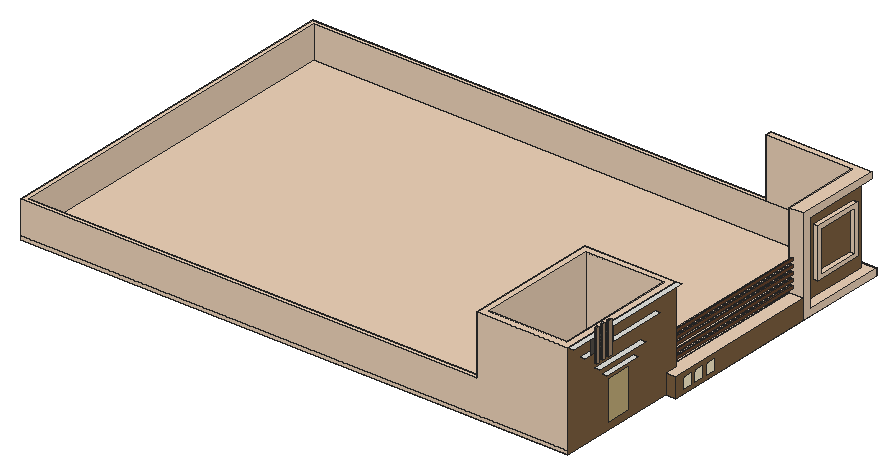
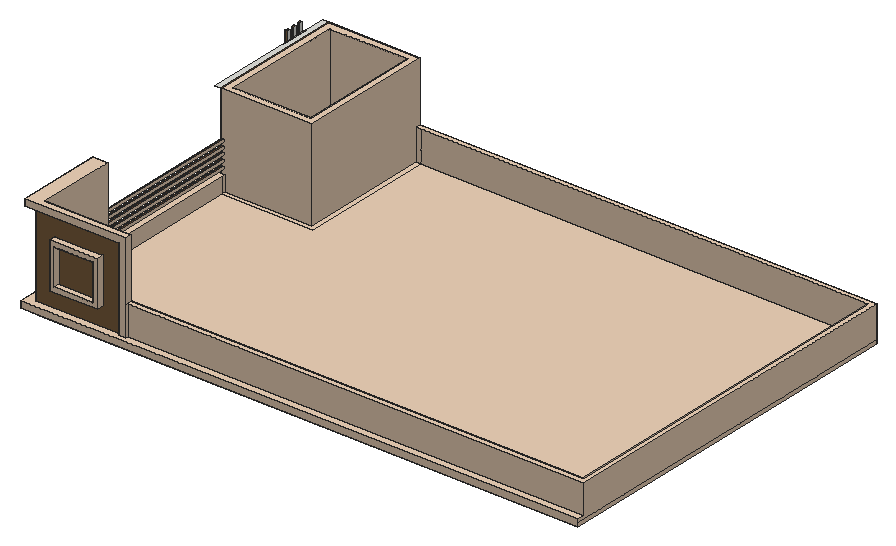
# SketchUp Ruby script. Lengths in inches.
U = 1.inch
M = Sketchup.active_model
def pt(a) = Geom::Point3d.new(a.map { |v| v * U })
def face(e, loops, mat)
  f = e.add_face(loops[0].map { |a| pt(a) })
  loops[1..].each { |l| e.add_face(l.map { |a| pt(a) }).erase! }
  f.material = f.back_material = mat if mat
  f
end
# faces: each face lists its corners as indices into pts; further lists are holes
def faces(e, pts, list, mat = nil) = list.each { |f| face(e, (f[0].is_a?(Array) ? f : [f]).map { |l| l.map { |i| pts[i] } }, mat) }
# xy, xz, yz: faces in a plane at the given z, y or x. An outline is a flat list of corners, or four numbers for a rectangle; further outlines are holes
def ring(l) = l.size == 4 ? [[l[0], l[1]], [l[2], l[1]], [l[2], l[3]], [l[0], l[3]]] : l.each_slice(2).to_a
def flat(e, list, mat, &to3) = list.each { |f| face(e, (f[0].is_a?(Array) ? f : [f]).map { |l| ring(l).map { |u, v| to3.(u, v) } }, mat) }
def xy(e, z, list, mat = nil) = flat(e, list, mat) { |x, y| [x, y, z] }
def xz(e, y, list, mat = nil) = flat(e, list, mat) { |x, z| [x, y, z] }
def yz(e, x, list, mat = nil) = flat(e, list, mat) { |y, z| [x, y, z] }
def lines(e, pts, list) = list.each { |a, b| e.add_line(pt(pts[a]), pt(pts[b])) }
# prism: a flat outline (further loops are holes) pulled along v
def prism(e, loops, v, mat = nil)
  f = face(e, loops, mat); d = Geom::Vector3d.new(v.map { |x| x * U })
  f.pushpull(f.normal.samedirection?(d) ? d.length : -d.length)
end
def box(e, o, s, mat = nil) = prism(e, [[o, [o[0] + s[0], o[1], o[2]], [o[0] + s[0], o[1] + s[1], o[2]], [o[0], o[1] + s[1], o[2]]]], [0, 0, s[2]], mat)
def at(x, y, z, deg = 0) = Geom::Transformation.translation(pt([x, y, z])) * Geom::Transformation.rotation(ORIGIN, Z_AXIS, deg.degrees)
def axes(o, x, y, z) = Geom::Transformation.new([*x, 0, *y, 0, *z, 0, *pt(o).to_a, 1])
def part(name) = M.definitions.add(name)
# library, detail: a bought-in or finely detailed component or shape, given as its bounding box
def library(name, o, s) = part(name).tap { |d| box(d.entities, o, s) }
def detail(e, o, s) = box(e.add_group.entities, o, s)
def put(e, d, t, mat = nil) = e.add_instance(d, t).tap { |i| i.material = mat if mat }
def group(e, t, mat = nil) = e.add_group.tap { |g| g.transformation = t; g.material = mat if mat }.entities
root = M.entities
M.materials.add("D01_Frost_White").color = [255, 242, 206]
M.materials.add("Metal_10_1K").color = [196, 175, 123]
M.materials.add("Plywood_01_1K").color = [125, 96, 64]
M.materials.add("Roofing_01_1K").color = [84, 79, 73]
M.materials.add("ThomThom - Beard1").color = [168, 140, 112]
M.materials.add("ThomThom - Complexion1").color = [237, 210, 184]
M.materials.add("Wood_Veneer_15_1K").color = [103, 69, 45]
c1 = library("Sphere Light\#5",[-2.19,-2.19,-2.19],[4.38,4.38,4.38])
c2 = library("Sphere Light\#3",[-2.0625,-2.0625,-2.0625],[4.125,4.125,4.125])
c3 = library("Sphere Light\#4",[-1.85,-1.85,-1.85],[3.7,3.7,3.7])
xy(root,298,[[0,0,0,489.76,708,489.76,708,480,615,480,615,177,720,177,720,471,733.2,471,733.2,160.5,720,160.5,720,0],[[615,177,615,480,708,480,708,471,720,471,720,177],[705.14,198.45,705.92,198.54,706.65,198.83,707.28,199.29,707.77,199.91,708.08,200.625,708.19,201.4,708.1,202.18,707.82,202.91,707.35,203.53,706.74,204.02,706.02,204.33,705.24,204.45,704.47,204.36,703.74,204.07,703.11,203.61,702.62,202.99,702.31,202.27,702.19,201.5,702.28,200.72,702.57,199.99,703.04,199.36,703.65,198.875,704.37,198.56],[642.95,198.45,643.73,198.54,644.46,198.83,645.09,199.29,645.58,199.91,645.89,200.625,646,201.4,645.92,202.18,645.63,202.91,645.16,203.53,644.55,204.02,643.83,204.33,643.06,204.45,642.28,204.36,641.55,204.07,640.92,203.61,640.43,202.99,640.12,202.27,640.01,201.5,640.09,200.72,640.38,199.99,640.85,199.36,641.46,198.875,642.18,198.56],[705.14,325.42,705.92,325.51,706.65,325.8,707.28,326.27,707.77,326.88,708.08,327.6,708.19,328.37,708.1,329.15,707.82,329.88,707.35,330.51,706.74,330.99,706.02,331.31,705.24,331.42,704.47,331.33,703.74,331.05,703.11,330.58,702.62,329.97,702.31,329.25,702.19,328.47,702.28,327.69,702.57,326.97,703.04,326.34,703.65,325.85,704.37,325.54],[705.14,448.71,705.92,448.8,706.65,449.08,707.28,449.55,707.77,450.16,708.08,450.88,708.19,451.66,708.1,452.43,707.82,453.16,707.35,453.79,706.74,454.28,706.02,454.59,705.24,454.71,704.47,454.62,703.74,454.33,703.11,453.86,702.62,453.25,702.31,452.53,702.19,451.76,702.28,450.98,702.57,450.25,703.04,449.62,703.65,449.13,704.37,448.82],[642.77,448.71,643.55,448.8,644.28,449.08,644.9,449.55,645.39,450.16,645.7,450.88,645.82,451.66,645.73,452.43,645.44,453.16,644.98,453.79,644.36,454.28,643.64,454.59,642.87,454.71,642.09,454.62,641.36,454.33,640.73,453.86,640.25,453.25,639.93,452.53,639.82,451.76,639.91,450.98,640.2,450.25,640.66,449.62,641.28,449.13,641.99,448.82],[642.77,325.42,643.55,325.51,644.28,325.8,644.9,326.27,645.39,326.88,645.7,327.6,645.82,328.37,645.73,329.15,645.44,329.88,644.98,330.51,644.36,330.99,643.64,331.31,642.87,331.42,642.09,331.33,641.36,331.05,640.73,330.58,640.25,329.97,639.93,329.25,639.82,328.47,639.91,327.69,640.2,326.97,640.66,326.34,641.28,325.85,641.99,325.54]],[708,471,720,480],[720,471,733.2,489.76],[708,480,720,489.76]],"ThomThom - Complexion1")
xy(root,299.82,[[642.77,325.42,641.99,325.54,641.28,325.85,640.66,326.34,640.2,326.97,639.91,327.69,639.82,328.47,639.93,329.25,640.25,329.97,640.73,330.58,641.36,331.05,642.09,331.33,642.87,331.42,643.64,331.31,644.36,330.99,644.98,330.51,645.44,329.88,645.73,329.15,645.82,328.37,645.7,327.6,645.39,326.88,644.9,326.27,644.28,325.8,643.55,325.51],[705.14,325.42,704.37,325.54,703.65,325.85,703.04,326.34,702.57,326.97,702.28,327.69,702.19,328.47,702.31,329.25,702.62,329.97,703.11,330.58,703.74,331.05,704.47,331.33,705.24,331.42,706.02,331.31,706.74,330.99,707.35,330.51,707.82,329.88,708.1,329.15,708.19,328.37,708.08,327.6,707.77,326.88,707.28,326.27,706.65,325.8,705.92,325.51],[642.77,448.71,641.99,448.82,641.28,449.13,640.66,449.62,640.2,450.25,639.91,450.98,639.82,451.76,639.93,452.53,640.25,453.25,640.73,453.86,641.36,454.33,642.09,454.62,642.87,454.71,643.64,454.59,644.36,454.28,644.98,453.79,645.44,453.16,645.73,452.43,645.82,451.66,645.7,450.88,645.39,450.16,644.9,449.55,644.28,449.08,643.55,448.8],[705.14,448.71,704.37,448.82,703.65,449.13,703.04,449.62,702.57,450.25,702.28,450.98,702.19,451.76,702.31,452.53,702.62,453.25,703.11,453.86,703.74,454.33,704.47,454.62,705.24,454.71,706.02,454.59,706.74,454.28,707.35,453.79,707.82,453.16,708.1,452.43,708.19,451.66,708.08,450.88,707.77,450.16,707.28,449.55,706.65,449.08,705.92,448.8]],"ThomThom - Complexion1")
xy(root,299.97,[[642.95,198.45,642.18,198.56,641.46,198.875,640.85,199.36,640.38,199.99,640.09,200.72,640.01,201.5,640.12,202.27,640.43,202.99,640.92,203.61,641.55,204.07,642.28,204.36,643.06,204.45,643.83,204.33,644.55,204.02,645.16,203.53,645.63,202.91,645.92,202.18,646,201.4,645.89,200.625,645.58,199.91,645.09,199.29,644.46,198.83,643.73,198.54]],"ThomThom - Complexion1")
xy(root,300.15,[[705.14,198.45,704.37,198.56,703.65,198.875,703.04,199.36,702.57,199.99,702.28,200.72,702.19,201.5,702.31,202.27,702.62,202.99,703.11,203.61,703.74,204.07,704.47,204.36,705.24,204.45,706.02,204.33,706.74,204.02,707.35,203.53,707.82,202.91,708.1,202.18,708.19,201.4,708.08,200.625,707.77,199.91,707.28,199.29,706.65,198.83,705.92,198.54]],"ThomThom - Complexion1")
xy(root,304,[[6,6,594,6,594,183,714,183,714,474,6,474],[594,6,600,6,600,177,714,177,714,183,594,183],[609,9,711,168]],"ThomThom - Complexion1")
xy(root,307,[[720,379.83,733.2,379.83,733.2,489.76,0,489.76,0,480,600,480,600,483,609,483,609,480,720,480]],"ThomThom - Complexion1")
xy(root,324.11,[[720,160.5,733.2,160.5,733.2,370.83,714,370.83,714,177,720,177]],"ThomThom - Complexion1")
xy(root,329.0625,[[720,401.89,727.15,466.9375]],"ThomThom - Complexion1")
xy(root,330.42,[[715.7,170.9375,718.66,370.83]],"ThomThom - Complexion1")
xy(root,331,[[633,480,696,488.28]],"ThomThom - Complexion1")
xy(root,333.95,[[715.7,170.9375,718.66,370.83]],"Wood_Veneer_15_1K")
xy(root,334,[[720,406.83,727.15,462]],"ThomThom - Complexion1")
xy(root,337,[[639,480,690,488.28]],"ThomThom - Complexion1")
xy(root,338.27,[[715.7,170.9375,718.66,370.83]],"ThomThom - Complexion1")
xy(root,341.81,[[715.7,170.9375,718.66,370.83]],"Wood_Veneer_15_1K")
xy(root,346,[[0,0,600,0,600,6,6,6,6,474,600,474,600,480,0,480]],"ThomThom - Complexion1")
xy(root,346.62,[[715.7,170.9375,718.66,370.83]],"ThomThom - Complexion1")
xy(root,350.15,[[715.7,170.9375,718.66,370.83]],"Wood_Veneer_15_1K")
xy(root,354.49,[[715.7,170.9375,718.66,370.83]],"ThomThom - Complexion1")
xy(root,358.02,[[715.7,170.9375,718.66,370.83]],"Wood_Veneer_15_1K")
xy(root,362.31,[[715.7,170.9375,718.66,370.83]],"ThomThom - Complexion1")
xy(root,365.84,[[715.7,170.9375,718.66,370.83]],"Wood_Veneer_15_1K")
xy(root,370,[[722,54,728,105]])
xy(root,382,[[722,42,728,117]])
xy(root,385,[[639,480,690,488.28]],"ThomThom - Complexion1")
xy(root,388,[[720,406.83,727.15,462]],"ThomThom - Complexion1")
xy(root,391,[[633,480,696,488.28]],"ThomThom - Complexion1")
xy(root,392.9375,[[720,401.89,727.15,466.9375]],"ThomThom - Complexion1")
xy(root,394,[[728,33.04,731,37.39],[728,43.39,731,47.22],[728,53.22,731,57.32]])
xy(root,406,[[722,18,728,141]])
xy(root,415,[[720,379.83,733.2,483],[609,480,720,483]],"ThomThom - Complexion1")
xy(root,424,[[720,0,728,177]])
xy(root,424,[[[600,0,720,177],[609,9,711,168]],[714,370.83,733.2,370.83,733.2,483,600,483,600,474,714,474]],"ThomThom - Complexion1")
xy(root,436,[[728,33.04,731,37.39],[728,43.39,731,47.22],[728,53.22,731,57.32]],"Plywood_01_1K")
xz(root,0,[[0,298,720,302.48],[0,302.48,720,302.48,720,424,600,424,600,346,0,346]],"ThomThom - Complexion1")
xz(root,6,[[6,304,594,346],[594,304,600,346]],"ThomThom - Complexion1")
xz(root,9,[[609,304,711,424]],"ThomThom - Complexion1")
xz(root,33.04,[[728,394,731,436]],"Plywood_01_1K")
xz(root,37.39,[[728,394,731,436]],"Plywood_01_1K")
xz(root,43.39,[[728,394,731,436]],"Plywood_01_1K")
xz(root,47.22,[[728,394,731,436]],"Plywood_01_1K")
xz(root,53.22,[[728,394,731,436]],"Plywood_01_1K")
xz(root,57.32,[[728,394,731,436]],"Plywood_01_1K")
xz(root,160.5,[[720,298,733.2,324.11]],"Plywood_01_1K")
xz(root,168,[[609,304,711,424]],"ThomThom - Complexion1")
xz(root,170.9375,[[715.7,330.42,718.66,333.95],[715.7,338.27,718.66,341.81],[715.7,346.62,718.66,350.15],[715.7,354.49,718.66,358.02],[715.7,362.31,718.66,365.84]],"ThomThom - Complexion1")
xz(root,177,[[600,304,600,424,720,424,720,324.11,714,324.11,714,304]],"ThomThom - Complexion1")
xz(root,370.83,[[[714,324.11,733.2,424],[715.7,362.31,718.66,365.84],[715.7,354.49,718.66,358.02],[715.7,346.62,718.66,350.15],[715.7,338.27,718.66,341.81],[715.7,330.42,718.66,333.95]]],"ThomThom - Complexion1")
xz(root,379.83,[[720,307,733.2,415]],"ThomThom - Complexion1")
xz(root,401.89,[[720,329.0625,727.15,392.9375]],"ThomThom - Complexion1")
xz(root,406.83,[[720,334,727.15,388]],"ThomThom - Complexion1")
xz(root,462,[[720,334,727.15,388]],"ThomThom - Complexion1")
xz(root,466.9375,[[720,329.0625,727.15,392.9375]],"ThomThom - Complexion1")
xz(root,474,[[6,304,714,346],[600,346,714,424]],"ThomThom - Complexion1")
xz(root,480,[[[609,307,720,415],[633,331,696,391]],[639,337,690,385]],"Plywood_01_1K")
xz(root,480,[[0,307,600,346]],"ThomThom - Complexion1")
xz(root,483,[[600,307,600,424,733.2,424,733.2,415,609,415,609,307]],"ThomThom - Complexion1")
xz(root,488.28,[[[633,331,696,391],[639,337,690,385]]],"ThomThom - Complexion1")
xz(root,489.76,[[0,298,733.2,307]],"ThomThom - Complexion1")
yz(root,0,[[0,298,489.76,302.48],[0,302.48,0,346,480,346,480,307,489.76,307,489.76,302.48]],"ThomThom - Complexion1")
yz(root,6,[[6,304,474,346]],"ThomThom - Complexion1")
yz(root,600,[[6,304,6,346,0,346,0,424,177,424,177,304],[480,307,483,346],[474,346,483,424]],"ThomThom - Complexion1")
yz(root,609,[[9,304,168,424],[480,307,483,415]],"ThomThom - Complexion1")
yz(root,633,[[480,331,488.28,391]],"ThomThom - Complexion1")
yz(root,639,[[480,337,488.28,385]],"ThomThom - Complexion1")
yz(root,690,[[480,337,488.28,385]],"ThomThom - Complexion1")
yz(root,696,[[480,331,488.28,391]],"ThomThom - Complexion1")
yz(root,711,[[9,304,168,424]],"ThomThom - Complexion1")
yz(root,714,[[177,304,183,324.11],[183,304,183,324.11,370.83,324.11,370.83,424,474,424,474,304]],"ThomThom - Complexion1")
yz(root,715.7,[[170.9375,330.42,370.83,333.95],[170.9375,338.27,370.83,341.81],[170.9375,346.62,370.83,350.15],[170.9375,354.49,370.83,358.02],[170.9375,362.31,370.83,365.84]],"ThomThom - Complexion1")
yz(root,718.66,[[170.9375,330.42,370.83,333.95],[170.9375,338.27,370.83,341.81],[170.9375,346.62,370.83,350.15],[170.9375,354.49,370.83,358.02],[170.9375,362.31,370.83,365.84]],"Wood_Veneer_15_1K")
yz(root,720,[[0,298,160.5,298,160.5,324.11,177,324.11,177,424,0,424],[[379.83,307,480,415],[401.89,329.0625,466.9375,392.9375]],[406.83,334,462,388]],"Plywood_01_1K")
yz(root,722,[[64,309.5,95,360]],"Metal_10_1K")
yz(root,727.15,[[[401.89,329.0625,466.9375,392.9375],[406.83,334,462,388]]],"ThomThom - Complexion1")
yz(root,728,[[33.04,394,37.39,406],[43.39,394,47.22,406],[53.22,394,57.32,406],[33.04,406,37.39,424],[43.39,406,47.22,424],
  [53.22,406,57.32,424],[33.04,424,37.39,436],[43.39,424,47.22,436],[53.22,424,57.32,436]])
yz(root,728,[[27.04,406,33.04,424],[37.39,406,43.39,424],[47.22,406,53.22,424],[57.32,406,63.32,424]],"Roofing_01_1K")
yz(root,731,[[33.04,394,37.39,436],[43.39,394,47.22,436],[53.22,394,57.32,436]],"ThomThom - Beard1")
yz(root,733.2,[[173.05,303.92,185.15,317.39],[191.37,303.92,203.46,317.39],[210.77,303.92,222.86,317.39]],"D01_Frost_White")
yz(root,733.2,[[[160.5,298,370.83,324.11],[173.05,303.92,185.15,317.39],[191.37,303.92,203.46,317.39],[210.77,303.92,222.86,317.39]]],"Plywood_01_1K")
yz(root,733.2,[[370.83,298,489.76,298,489.76,307,379.83,307,379.83,415,483,415,483,424,370.83,424]],"ThomThom - Complexion1")
p = [[642.95,198.45,298],[642.18,198.56,298],[642.18,198.56,299.97],[642.95,198.45,299.97],[643.73,198.54,298],[643.73,198.54,299.97],
  [705.14,198.45,298],[704.37,198.56,298],[704.37,198.56,300.15],[705.14,198.45,300.15],[705.92,198.54,298],[705.92,198.54,300.15],
  [644.46,198.83,298],[644.46,198.83,299.97],[706.65,198.83,298],[706.65,198.83,300.15],[641.46,198.875,298],[641.46,198.875,299.97],
  [703.65,198.875,298],[703.65,198.875,300.15],[645.09,199.29,298],[645.09,199.29,299.97],[707.28,199.29,298],[707.28,199.29,300.15],
  [640.85,199.36,298],[640.85,199.36,299.97],[703.04,199.36,298],[703.04,199.36,300.15],[645.58,199.91,298],[645.58,199.91,299.97],
  [707.77,199.91,298],[707.77,199.91,300.15],[640.38,199.99,298],[640.38,199.99,299.97],[702.57,199.99,298],[702.57,199.99,300.15],
  [645.89,200.625,298],[645.89,200.625,299.97],[708.08,200.625,298],[708.08,200.625,300.15],[640.09,200.72,298],[640.09,200.72,299.97],
  [702.28,200.72,298],[702.28,200.72,300.15],[646,201.4,298],[646,201.4,299.97],[708.19,201.4,298],[708.19,201.4,300.15],
  [640.01,201.5,298],[640.01,201.5,299.97],[702.19,201.5,298],[702.19,201.5,300.15],[645.92,202.18,298],[645.92,202.18,299.97],
  [708.1,202.18,298],[708.1,202.18,300.15],[640.12,202.27,298],[640.12,202.27,299.97],[702.31,202.27,298],[702.31,202.27,300.15],
  [645.63,202.91,298],[645.63,202.91,299.97],[707.82,202.91,298],[707.82,202.91,300.15],[640.43,202.99,298],[640.43,202.99,299.97],
  [702.62,202.99,298],[702.62,202.99,300.15],[645.16,203.53,298],[645.16,203.53,299.97],[707.35,203.53,298],[707.35,203.53,300.15],
  [640.92,203.61,298],[640.92,203.61,299.97],[703.11,203.61,298],[703.11,203.61,300.15],[644.55,204.02,298],[644.55,204.02,299.97],
  [706.74,204.02,298],[706.74,204.02,300.15],[641.55,204.07,298],[641.55,204.07,299.97],[703.74,204.07,298],[703.74,204.07,300.15],
  [643.83,204.33,298],[643.83,204.33,299.97],[706.02,204.33,298],[706.02,204.33,300.15],[642.28,204.36,298],[642.28,204.36,299.97],
  [704.47,204.36,298],[704.47,204.36,300.15],[643.06,204.45,298],[643.06,204.45,299.97],[705.24,204.45,298],[705.24,204.45,300.15],
  [642.77,325.42,298],[641.99,325.54,298],[641.99,325.54,299.82],[642.77,325.42,299.82],[643.55,325.51,298],[643.55,325.51,299.82],
  [705.14,325.42,298],[704.37,325.54,298],[704.37,325.54,299.82],[705.14,325.42,299.82],[705.92,325.51,298],[705.92,325.51,299.82],
  [641.28,325.85,298],[641.28,325.85,299.82],[644.28,325.8,298],[644.28,325.8,299.82],[703.65,325.85,298],[703.65,325.85,299.82],
  [706.65,325.8,298],[706.65,325.8,299.82],[640.66,326.34,298],[640.66,326.34,299.82],[644.9,326.27,298],[644.9,326.27,299.82],
  [703.04,326.34,298],[703.04,326.34,299.82],[707.28,326.27,298],[707.28,326.27,299.82],[640.2,326.97,298],[640.2,326.97,299.82],
  [645.39,326.88,298],[645.39,326.88,299.82],[702.57,326.97,298],[702.57,326.97,299.82],[707.77,326.88,298],[707.77,326.88,299.82],
  [645.7,327.6,298],[645.7,327.6,299.82],[708.08,327.6,298],[708.08,327.6,299.82],[639.91,327.69,298],[639.91,327.69,299.82],
  [702.28,327.69,298],[702.28,327.69,299.82],[645.82,328.37,298],[645.82,328.37,299.82],[708.19,328.37,298],[708.19,328.37,299.82],
  [639.82,328.47,298],[639.82,328.47,299.82],[702.19,328.47,298],[702.19,328.47,299.82],[645.73,329.15,298],[645.73,329.15,299.82],
  [708.1,329.15,298],[708.1,329.15,299.82],[639.93,329.25,298],[639.93,329.25,299.82],[702.31,329.25,298],[702.31,329.25,299.82],
  [645.44,329.88,298],[645.44,329.88,299.82],[707.82,329.88,298],[707.82,329.88,299.82],[640.25,329.97,298],[640.25,329.97,299.82],
  [702.62,329.97,298],[702.62,329.97,299.82],[644.98,330.51,298],[644.98,330.51,299.82],[707.35,330.51,298],[707.35,330.51,299.82],
  [640.73,330.58,298],[640.73,330.58,299.82],[703.11,330.58,298],[703.11,330.58,299.82],[644.36,330.99,298],[644.36,330.99,299.82],
  [706.74,330.99,298],[706.74,330.99,299.82],[641.36,331.05,298],[641.36,331.05,299.82],[703.74,331.05,298],[703.74,331.05,299.82],
  [642.09,331.33,298],[642.09,331.33,299.82],[643.64,331.31,298],[643.64,331.31,299.82],[704.47,331.33,298],[704.47,331.33,299.82],
  [706.02,331.31,298],[706.02,331.31,299.82],[642.87,331.42,298],[642.87,331.42,299.82],[705.24,331.42,298],[705.24,331.42,299.82],
  [642.77,448.71,298],[641.99,448.82,298],[641.99,448.82,299.82],[642.77,448.71,299.82],[643.55,448.8,298],[643.55,448.8,299.82],
  [705.14,448.71,298],[704.37,448.82,298],[704.37,448.82,299.82],[705.14,448.71,299.82],[705.92,448.8,298],[705.92,448.8,299.82],
  [641.28,449.13,298],[641.28,449.13,299.82],[644.28,449.08,298],[644.28,449.08,299.82],[703.65,449.13,298],[703.65,449.13,299.82],
  [706.65,449.08,298],[706.65,449.08,299.82],[640.66,449.62,298],[640.66,449.62,299.82],[644.9,449.55,298],[644.9,449.55,299.82],
  [703.04,449.62,298],[703.04,449.62,299.82],[707.28,449.55,298],[707.28,449.55,299.82],[645.39,450.16,298],[645.39,450.16,299.82],
  [707.77,450.16,298],[707.77,450.16,299.82],[640.2,450.25,298],[640.2,450.25,299.82],[702.57,450.25,298],[702.57,450.25,299.82],
  [639.91,450.98,298],[639.91,450.98,299.82],[645.7,450.88,298],[645.7,450.88,299.82],[702.28,450.98,298],[702.28,450.98,299.82],
  [708.08,450.88,298],[708.08,450.88,299.82],[645.82,451.66,298],[645.82,451.66,299.82],[708.19,451.66,298],[708.19,451.66,299.82],
  [639.82,451.76,298],[639.82,451.76,299.82],[702.19,451.76,298],[702.19,451.76,299.82],[645.73,452.43,298],[645.73,452.43,299.82],
  [708.1,452.43,298],[708.1,452.43,299.82],[639.93,452.53,298],[639.93,452.53,299.82],[702.31,452.53,298],[702.31,452.53,299.82],
  [645.44,453.16,298],[645.44,453.16,299.82],[707.82,453.16,298],[707.82,453.16,299.82],[640.25,453.25,298],[640.25,453.25,299.82],
  [702.62,453.25,298],[702.62,453.25,299.82],[640.73,453.86,298],[640.73,453.86,299.82],[644.98,453.79,298],[644.98,453.79,299.82],
  [703.11,453.86,298],[703.11,453.86,299.82],[707.35,453.79,298],[707.35,453.79,299.82],[644.36,454.28,298],[644.36,454.28,299.82],
  [706.74,454.28,298],[706.74,454.28,299.82],[641.36,454.33,298],[641.36,454.33,299.82],[703.74,454.33,298],[703.74,454.33,299.82],
  [642.09,454.62,298],[642.09,454.62,299.82],[643.64,454.59,298],[643.64,454.59,299.82],[704.47,454.62,298],[704.47,454.62,299.82],
  [706.02,454.59,298],[706.02,454.59,299.82],[642.87,454.71,298],[642.87,454.71,299.82],[705.24,454.71,298],[705.24,454.71,299.82],
  [720,423.06,302],[720,423.06,298],[714,474,338.18],[714,480,338.18],[714,474,330.3125],[714,480,330.3125],
  [714,474,321.97],[714,480,321.97],[714,474,314.11],[714,480,314.11],[720,471,307],[711,480,313]]
faces(root,p,[[0,1,2,3],[4,0,3,5],[6,7,8,9],[10,6,9,11],[12,4,5,13],[14,10,11,15],[1,16,17,2],[7,18,19,8],
  [20,12,13,21],[22,14,15,23],[16,24,25,17],[18,26,27,19],[28,20,21,29],[30,22,23,31],[24,32,33,25],[26,34,35,27],
  [36,28,29,37],[38,30,31,39],[32,40,41,33],[34,42,43,35],[44,36,37,45],[46,38,39,47],[40,48,49,41],[42,50,51,43],
  [52,44,45,53],[54,46,47,55],[48,56,57,49],[50,58,59,51],[60,52,53,61],[62,54,55,63],[56,64,65,57],[58,66,67,59],
  [68,60,61,69],[70,62,63,71],[64,72,73,65],[66,74,75,67],[76,68,69,77],[78,70,71,79],[72,80,81,73],[74,82,83,75],
  [84,76,77,85],[86,78,79,87],[80,88,89,81],[82,90,91,83],[92,84,85,93],[94,86,87,95],[88,92,93,89],[90,94,95,91],
  [96,97,98,99],[100,96,99,101],[102,103,104,105],[106,102,105,107],[97,108,109,98],[110,100,101,111],[103,112,113,104],[114,106,107,115],
  [108,116,117,109],[118,110,111,119],[112,120,121,113],[122,114,115,123],[116,124,125,117],[126,118,119,127],[120,128,129,121],[130,122,123,131],
  [132,126,127,133],[134,130,131,135],[124,136,137,125],[128,138,139,129],[140,132,133,141],[142,134,135,143],[136,144,145,137],[138,146,147,139],
  [148,140,141,149],[150,142,143,151],[144,152,153,145],[146,154,155,147],[156,148,149,157],[158,150,151,159],[152,160,161,153],[154,162,163,155],
  [164,156,157,165],[166,158,159,167],[160,168,169,161],[162,170,171,163],[172,164,165,173],[174,166,167,175],[168,176,177,169],[170,178,179,171],
  [176,180,181,177],[182,172,173,183],[178,184,185,179],[186,174,175,187],[180,188,189,181],[188,182,183,189],[184,190,191,185],[190,186,187,191],
  [192,193,194,195],[196,192,195,197],[198,199,200,201],[202,198,201,203],[193,204,205,194],[206,196,197,207],[199,208,209,200],[210,202,203,211],
  [204,212,213,205],[214,206,207,215],[208,216,217,209],[218,210,211,219],[220,214,215,221],[222,218,219,223],[212,224,225,213],[216,226,227,217],
  [224,228,229,225],[230,220,221,231],[226,232,233,227],[234,222,223,235],[236,230,231,237],[238,234,235,239],[228,240,241,229],[232,242,243,233],
  [244,236,237,245],[246,238,239,247],[240,248,249,241],[242,250,251,243],[252,244,245,253],[254,246,247,255],[248,256,257,249],[250,258,259,251],
  [256,260,261,257],[262,252,253,263],[258,264,265,259],[266,254,255,267],[268,262,263,269],[270,266,267,271],[260,272,273,261],[264,274,275,265],
  [272,276,277,273],[278,268,269,279],[274,280,281,275],[282,270,271,283],[276,284,285,277],[284,278,279,285],[280,286,287,281],[286,282,283,287]],"ThomThom - Complexion1")
lines(root,p,[[288,289],[290,291],[292,293],[294,295],[296,297],[298,299]])
put(root,c1,at(642.68,451.65,299.82),"ThomThom - Complexion1")
put(root,c2,at(642.91,328.41,299.82),"ThomThom - Complexion1")
put(root,c3,at(705.35,451.64,299.82),"ThomThom - Complexion1")
